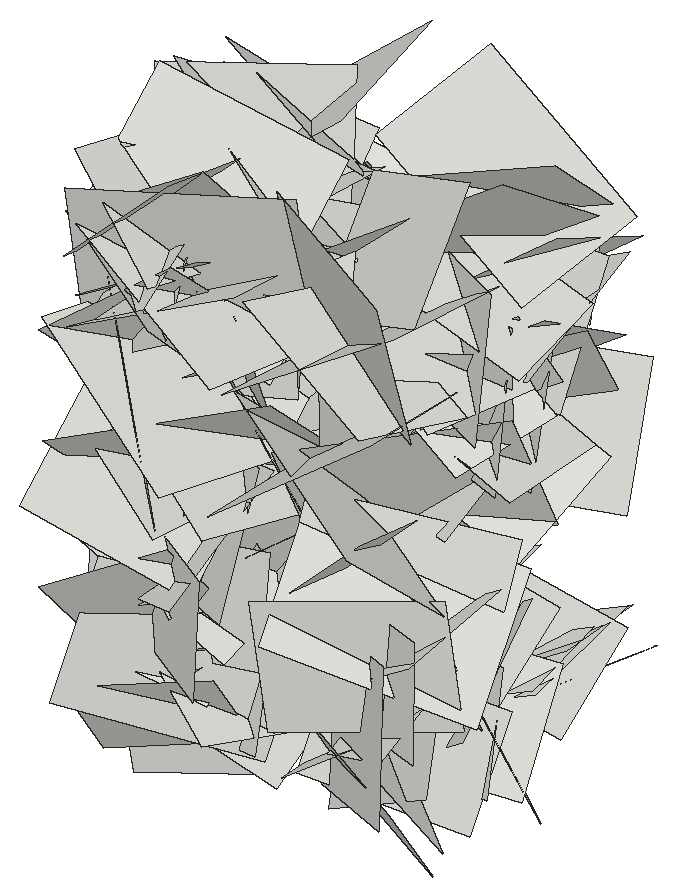
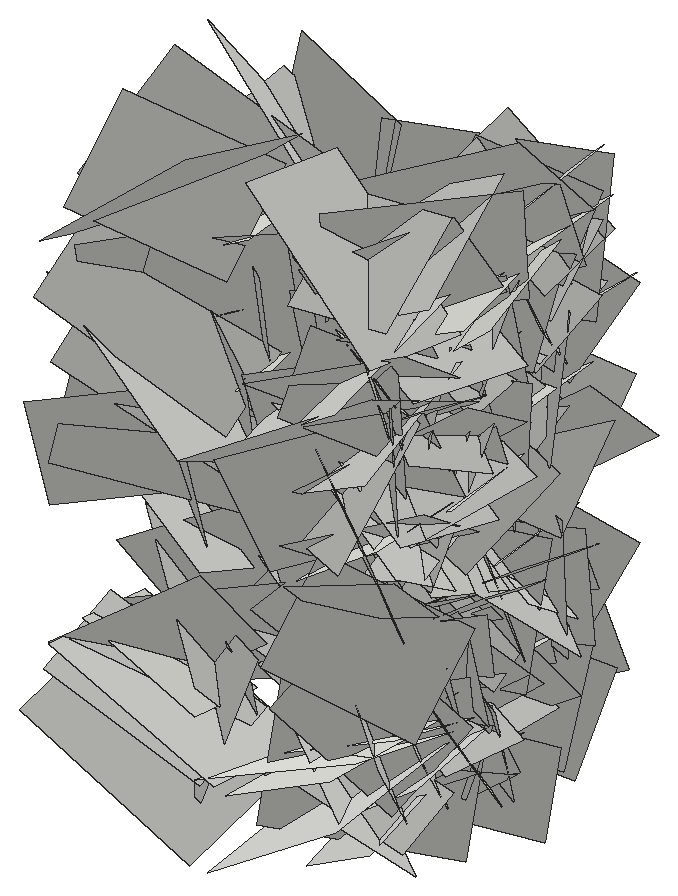
# SketchUp Ruby script. Lengths in inches.
U = 1.inch
M = Sketchup.active_model
def pt(a) = Geom::Point3d.new(a.map { |v| v * U })
def face(e, loops, mat)
  f = e.add_face(loops[0].map { |a| pt(a) })
  loops[1..].each { |l| e.add_face(l.map { |a| pt(a) }).erase! }
  f.material = f.back_material = mat if mat
  f
end
# faces: each face lists its corners as indices into pts; further lists are holes
def faces(e, pts, list, mat = nil) = list.each { |f| face(e, (f[0].is_a?(Array) ? f : [f]).map { |l| l.map { |i| pts[i] } }, mat) }
# xy, xz, yz: faces in a plane at the given z, y or x. An outline is a flat list of corners, or four numbers for a rectangle; further outlines are holes
def ring(l) = l.size == 4 ? [[l[0], l[1]], [l[2], l[1]], [l[2], l[3]], [l[0], l[3]]] : l.each_slice(2).to_a
def flat(e, list, mat, &to3) = list.each { |f| face(e, (f[0].is_a?(Array) ? f : [f]).map { |l| ring(l).map { |u, v| to3.(u, v) } }, mat) }
def xy(e, z, list, mat = nil) = flat(e, list, mat) { |x, y| [x, y, z] }
def xz(e, y, list, mat = nil) = flat(e, list, mat) { |x, z| [x, y, z] }
def yz(e, x, list, mat = nil) = flat(e, list, mat) { |y, z| [x, y, z] }
def lines(e, pts, list) = list.each { |a, b| e.add_line(pt(pts[a]), pt(pts[b])) }
# prism: a flat outline (further loops are holes) pulled along v
def prism(e, loops, v, mat = nil)
  f = face(e, loops, mat); d = Geom::Vector3d.new(v.map { |x| x * U })
  f.pushpull(f.normal.samedirection?(d) ? d.length : -d.length)
end
def box(e, o, s, mat = nil) = prism(e, [[o, [o[0] + s[0], o[1], o[2]], [o[0] + s[0], o[1] + s[1], o[2]], [o[0], o[1] + s[1], o[2]]]], [0, 0, s[2]], mat)
def at(x, y, z, deg = 0) = Geom::Transformation.translation(pt([x, y, z])) * Geom::Transformation.rotation(ORIGIN, Z_AXIS, deg.degrees)
def axes(o, x, y, z) = Geom::Transformation.new([*x, 0, *y, 0, *z, 0, *pt(o).to_a, 1])
def part(name) = M.definitions.add(name)
# library, detail: a bought-in or finely detailed component or shape, given as its bounding box
def library(name, o, s) = part(name).tap { |d| box(d.entities, o, s) }
def detail(e, o, s) = box(e.add_group.entities, o, s)
def put(e, d, t, mat = nil) = e.add_instance(d, t).tap { |i| i.material = mat if mat }
def group(e, t, mat = nil) = e.add_group.tap { |g| g.transformation = t; g.material = mat if mat }.entities
root = M.entities
c1 = part("Component\#6")
p = [[0.01,0,0],[0,3.24,4.54],[4.32,3.24,4.54],[4.33,0,0]]
faces(c1.entities,p,[[0,1,2,3]])
put(root,c1,axes([24.34,192.1875,23.6],[0.04344,0.89705,-0.17333],[-0.1764,-0.16328,-0.88435],[0.95226,-0.07116,-0.15591]))
put(root,c1,axes([28.31,192.1875,23.6],[-0.04344,0.89705,-0.17333],[0.1764,-0.16328,-0.88435],[-0.95226,-0.07116,-0.15591]))
put(root,c1,axes([24.34,200.85,9.74],[0.02518,0.49854,0.49521],[0.19267,0.47427,-0.48618],[0.7195,-0.14445,0.11286]))
put(root,c1,axes([28.31,200.46,4.14],[-0.03987,0.66432,-0.22968],[-0.12809,-0.2327,-0.65325],[-0.73398,0.00452,0.12648]))
put(root,c1,axes([24.34,196.11,19.5625],[-0.1708,0.27531,1.11719],[-0.21419,1.10379,-0.30115],[1.2007,0.23607,0.1052]))
put(root,c1,axes([24.34,195.27,-1.16],[-0.10176,-0.07093,0.82892],[0.16666,0.81783,0.08819],[0.86597,-0.16573,0.08043]))
put(root,c1,axes([28.31,202.11,15.27],[-0.00741,-0.76642,-0.19435],[-0.02033,-0.19414,0.76626],[-0.83787,0.01149,-0.01688]))
put(root,c1,axes([28.31,201.99,11.3125],[0.07595,0.62186,-0.76254],[0.14567,-0.76339,-0.60964],[-1.03278,-0.06194,-0.14206]))
put(root,c1,axes([24.34,202.38,16.09],[-0.07402,-0.92988,-0.45649],[-0.17154,-0.44211,0.92536],[1.08456,-0.13339,0.1152]))
put(root,c1,axes([24.34,193.92,18.08],[-0.13809,0.41624,-1.10581],[-0.27382,-1.09563,-0.38198],[1.22215,-0.19844,-0.21052]))
put(root,c1,axes([28.31,193.9,23.36],[-0.05376,0.55183,-0.55937],[0.04326,-0.55793,-0.55411],[-0.83178,-0.06469,0.00734]))
put(root,c1,axes([24.34,196.25,20.97],[0.03433,0.46285,-0.75346],[-0.09275,-0.74858,-0.46362],[0.93272,-0.09148,-0.01837]))
put(root,c1,axes([24.34,193.09,19.46],[0.07295,0.25641,0.83596],[-0.12348,0.83376,-0.24615],[0.9186,0.09171,-0.09948]))
put(root,c1,axes([28.31,200.69,6.875],[0.16125,-0.91938,-0.30199],[0.04119,-0.29965,0.93182],[-1.02494,-0.15668,-0.01006]))
put(root,c1,axes([24.34,194.43,21.03],[-0.18864,1.08922,-0.2367],[-0.12278,-0.25647,-1.09312],[1.17512,0.14806,-0.15221]))
put(root,c1,axes([24.34,195.95,14.86],[-0.17446,0.9838,0.62037],[-0.19333,0.59697,-0.99508],[1.2176,0.23574,-0.06911]))
put(root,c1,axes([24.34,200.41,3.58],[-0.05776,-0.87144,-0.04483],[0.06577,-0.04867,0.87073],[0.92261,-0.05109,-0.06488]))
put(root,c1,axes([24.34,198.3125,4.47],[-0.08144,0.93817,-0.09306],[-0.01009,-0.09413,-0.94116],[0.99929,0.07551,-0.01709]))
put(root,c1,axes([24.34,200.05,13.66],[0.07814,0.81604,-0.08962],[-0.02759,-0.08761,-0.81916],[0.86976,-0.0761,-0.01794]))
put(root,c1,axes([24.34,196.375,20.79],[-0.12547,0.87042,-0.10702],[0.18806,-0.08199,-0.86307],[0.91037,0.1369,0.16354]))
put(root,c1,axes([24.34,195.73,16.63],[-0.01219,-0.78698,0.32297],[0.05977,0.32158,0.78561],[0.89973,-0.03203,-0.04781]))
put(root,c1,axes([28.31,200.82,0.59],[-0.02153,-0.73416,-0.35765],[0.0933,-0.35764,0.72915],[-0.8606,-0.02041,0.08799]))
put(root,c1,axes([24.34,193.46,10.77],[0.10152,0.90556,-0.18731],[-0.17799,-0.16815,-0.89879],[0.96391,-0.12642,-0.14624]))
put(root,c1,axes([24.34,196.17,12.88],[-0.06274,0.02618,0.84664],[0.15393,0.83645,-0.01571],[0.88457,-0.1437,0.06278]))
put(root,c1,axes([24.34,195.4375,18.11],[0.16874,-0.51977,-0.57708],[-0.05885,-0.59519,0.52076],[0.82114,0.06415,0.15591]))
put(root,c1,axes([28.31,195.9375,9.16],[-0.07841,0.69576,-0.29748],[0.09095,-0.28926,-0.69787],[-0.79692,-0.10147,-0.05038]))
put(root,c1,axes([24.34,198.67,11.97],[-0.07539,0.76068,0.50866],[0.0723,0.51318,-0.75791],[0.96729,0.02092,0.0963]))
put(root,c1,axes([28.31,195.99,4.23],[0.18601,0.0566,0.88651],[-0.05201,0.90288,-0.04793],[-0.94017,-0.03875,0.17804]))
put(root,c1,axes([28.31,197.35,3.52],[-0.03443,0.41092,0.66217],[0.08038,0.66126,-0.40665],[-0.82215,0.04744,-0.06748]))
put(root,c1,axes([24.34,192.22,20.81],[0.00161,0.62306,-0.59539],[0.0785,-0.59329,-0.62067],[0.91013,0.05007,0.05459]))
put(root,c1,axes([28.31,202.74,-0.14],[-0.03158,-0.64507,0.25861],[-0.01592,0.25938,0.64528],[-0.73651,0.02205,-0.02503]))
put(root,c1,axes([24.34,195.86,16.68],[0.06531,-0.43873,0.684],[0.07025,0.68639,0.43429],[0.8585,-0.02279,-0.08757]))
put(root,c1,axes([28.31,202.51,19.98],[-0.06792,0.48446,-0.5602],[0.10116,-0.55221,-0.48846],[-0.77852,-0.11402,-0.01459]))
put(root,c1,axes([28.31,192.04,10.01],[0.12172,0.5206,-0.6372],[-0.01939,-0.6416,-0.52749],[-0.87198,0.08694,-0.07722]))
put(root,c1,axes([28.31,198.38,4.95],[0.02223,0.32868,-0.55446],[-0.17267,-0.53404,-0.32274],[-0.66105,0.15055,0.06565]))
put(root,c1,axes([24.34,199.37,10.67],[-0.09558,-1.01864,0.46326],[-0.13943,0.47118,1.01047],[1.17795,-0.02688,0.1572]))
put(root,c1,axes([28.31,192.95,10.8],[-0.02962,0.02518,0.78508],[0.12702,0.77652,-0.02064],[-0.82287,0.11896,-0.03145]))
put(root,c1,axes([28.31,200.03,9.27],[0.00412,-0.60297,0.30435],[-0.07057,0.30253,0.60022],[-0.71247,-0.03345,-0.05769]))
put(root,c1,axes([28.31,199.6875,17.84],[-0.07891,0.44569,0.39814],[-0.07493,0.39183,-0.45185],[-0.62903,-0.10259,0.00388]))
put(root,c1,axes([28.31,200.4375,8.06],[0.17377,0.75884,-0.49804],[0.05898,-0.51355,-0.76415],[-0.96033,0.10576,-0.13705]))
put(root,c1,axes([28.31,195.68,15.75],[-0.06715,-0.51242,0.33521],[-0.05381,0.34023,0.51051],[-0.64683,0.02489,-0.07727]))
put(root,c1,axes([28.31,198.91,12.75],[0.15355,-0.10183,1.00426],[0.21738,0.99636,0.07145],[-1.04766,0.19182,0.16201]))
put(root,c1,axes([28.31,196.5625,6.92],[-0.07674,-0.09799,-0.6482],[0.03176,-0.65195,0.09521],[-0.69417,-0.019,0.07601]))
put(root,c1,axes([28.31,199.23,1.1],[0.00098,-0.71414,-0.15761],[0.04174,-0.15733,0.71311],[-0.77408,-0.00939,0.03826]))
put(root,c1,axes([28.31,192.26,20.51],[0.14395,0.6641,-0.62024],[0.10915,-0.63433,-0.65665],[-0.95701,0.02754,-0.16819]))
put(root,c1,axes([28.31,193.91,15.9375],[-0.03263,0.61645,-0.26034],[0.02336,-0.25954,-0.61716],[-0.70894,-0.03692,-0.00835]))
put(root,c1,axes([28.31,202.9,8.46],[0.28421,-0.45126,-0.90988],[0.10984,-0.92399,0.48879],[-1.07096,-0.21452,-0.19133]))
put(root,c1,axes([24.34,199.68,18.17],[-0.10811,0.81171,0.57509],[0.11351,0.5837,-0.80488],[1.04835,0.0205,0.14645]))
put(root,c1,axes([28.31,193.57,4.75],[-0.0218,0.6351,0.02763],[-0.03876,0.02642,-0.63443],[-0.67273,-0.0221,0.03566]))
put(root,c1,axes([24.34,189.31,11.46],[0.01967,0.80876,0.77653],[-0.21901,0.76581,-0.79265],[1.16812,0.12996,-0.16169]))
put(root,c1,axes([24.34,202.76,13.17],[-0.11284,-1.03894,-0.17524],[0.03066,-0.17895,1.04335],[1.11641,-0.1001,-0.04636]))
put(root,c1,axes([28.31,195.85,11.01],[0.15114,0.73817,0.19544],[-0.07767,0.21113,-0.74396],[-0.80568,0.11812,0.10838]))
put(root,c1,axes([28.31,190.79,19.57],[-0.04866,0.55121,0.30162],[-0.00575,0.30207,-0.55285],[-0.66601,-0.04288,-0.01726]))
put(root,c1,axes([24.34,196.07,8.125],[0.08332,-0.69698,-0.457],[0.10667,-0.44773,0.70016],[0.87699,0.12068,-0.04174]))
put(root,c1,axes([28.31,199.64,2.06],[0.21894,0.61345,0.59822],[-0.01858,0.61825,-0.62794],[-0.90807,0.13525,0.15708]))
put(root,c1,axes([28.31,202.56,19.21],[-0.06396,-0.26998,-0.58675],[0.04641,-0.58965,0.26682],[-0.68306,-0.01478,0.07307]))
put(root,c1,axes([24.34,197.24,20.32],[0.11105,0.4932,0.81979],[-0.10012,0.82599,-0.48487],[1.00916,0.02768,-0.13831]))
put(root,c1,axes([24.34,196.19,13.89],[-0.03711,0.95345,-0.08325],[0.1071,-0.07916,-0.94908],[1.00884,0.04348,0.09769]))
put(root,c1,axes([28.31,198.53,13.8],[0.10676,-0.41647,0.70694],[0.09382,0.7136,0.40779],[-0.86465,0.02601,0.13154]))
put(root,c1,axes([28.31,201.03,8.02],[0.03451,-0.61291,-0.20918],[-0.0475,-0.21108,0.61149],[-0.68484,-0.01625,-0.05296]))
put(root,c1,axes([28.31,199.53,17.66],[0.07108,0.22718,0.77768],[0.14032,0.76678,-0.23541],[-0.84726,0.14605,0.02626]))
put(root,c1,axes([28.31,196.1,5.28],[0.08762,-0.56519,-0.39893],[-0.0287,-0.4041,0.56691],[-0.73275,-0.05175,-0.06991]))
put(root,c1,axes([24.34,192.44,8.79],[-0.05887,1.04295,0.25043],[0.00297,0.2509,-1.04431],[1.13694,0.05335,0.0157]))
put(root,c1,axes([24.34,193.71,0.46],[0.00413,-0.52236,0.7551],[0.18121,0.74232,0.51263],[0.95624,-0.13842,-0.10041]))
put(root,c1,axes([24.34,195.28,4.79],[0.03702,0.87634,0.85063],[-0.28559,0.83554,-0.84973],[1.26267,0.16329,-0.21713]))
put(root,c1,axes([24.34,203.91,5.3125],[0.18463,-0.58129,-0.78091],[-0.13848,-0.80009,0.56643],[1.02258,-0.00339,0.2177]))
put(root,c1,axes([24.34,198.93,5.125],[0.08676,0.85287,0.14934],[0.16568,0.13299,-0.84515],[0.90272,-0.10637,0.14076]))
put(root,c1,axes([24.34,198.84,9.75],[-0.24721,-0.9594,-0.88495],[-0.06038,-0.89063,0.98057],[1.38221,-0.2105,-0.11544]))
put(root,c1,axes([24.34,202.1,18.26],[-0.1919,-1.13475,-0.09678],[0.16378,-0.12156,1.13628],[1.19604,-0.16542,-0.17113]))
put(root,c1,axes([28.31,194.11,10.49],[0.01019,-0.66626,0.06574],[0.1187,0.06642,0.65679],[-0.69967,0.00157,0.11238]))
put(root,c1,axes([24.34,200.51,5.45],[-0.07717,-0.59417,-0.91785],[0.09928,-0.91989,0.58806],[1.15472,0.03938,-0.1119]))
put(root,c1,axes([24.34,205.24,14.9],[-0.1168,-0.46047,-1.13614],[-0.0362,-1.13913,0.465],[1.29896,-0.07315,-0.0892]))
put(root,c1,axes([24.34,194.25,1.05],[0.1707,-0.55728,0.79671],[-0.04122,0.80323,0.5697],[1.02978,0.12452,-0.10926]))
put(root,c1,axes([24.34,194.35,10.5],[-0.1187,0.07765,-1.12146],[0.14385,-1.11784,-0.09095],[1.18288,0.14373,-0.10148]))
put(root,c1,axes([24.34,197.36,24.8],[-0.09794,1.0389,-0.68546],[-0.01654,-0.68826,-1.04104],[1.31923,0.0685,-0.06394]))
put(root,c1,axes([28.31,199.74,12.37],[0.13977,-0.41949,-0.41774],[-0.0557,-0.43458,0.41982],[-0.62506,-0.05508,-0.13082]))
put(root,c1,axes([28.31,199.42,15.6],[0.03605,-0.49998,-0.38134],[0.14474,-0.36691,0.49324],[-0.65063,-0.10932,0.0886]))
put(root,c1,axes([24.34,200.08,24.34],[0.03463,0.75517,-0.67877],[0.20748,-0.67107,-0.73718],[1.05612,0.10708,0.16708]))
put(root,c1,axes([24.34,199.09,16.39],[0.13116,-1.14374,0.05938],[-0.13174,0.04596,1.1443],[1.20683,0.12933,0.11846]))
put(root,c1,axes([24.34,192.66,5.0625],[0.03803,0.06475,1.02957],[0.25075,1.00223,-0.07127],[1.06436,-0.23842,-0.02]))
put(root,c1,axes([24.34,196.53,2.03],[0.14871,0.38131,0.94323],[0.09041,0.94439,-0.39446],[1.07463,-0.13222,-0.09734]))
put(root,c1,axes([24.34,200.2,14.91],[0.20407,-0.96139,-0.18597],[0.07393,-0.17559,0.97991],[1.03533,0.20204,-0.03331]))
put(root,c1,axes([24.34,198.375,11.05],[-0.00636,-0.47599,-1.14741],[-0.03555,-1.14695,0.47597],[1.31628,-0.03327,0.00731]))
put(root,c1,axes([24.34,202.25,12.93],[-0.19135,-1.27912,0.12446],[0.2118,0.09622,1.27869],[1.34571,-0.19703,-0.18355]))
put(root,c1,axes([24.34,197.86,18.23],[0.19608,0.2602,-1.0463],[-0.01915,-1.06069,-0.26697],[1.14269,-0.06243,0.17507]))
put(root,c1,axes([24.34,197.84,4.84],[0.11369,-0.36766,-0.96616],[0.19069,-0.94989,0.38144],[1.07906,0.2066,0.03439]))
put(root,c1,axes([24.34,200.375,7.61],[0.26418,-0.51362,-0.84712],[0.05211,-0.86603,0.53955],[1.04881,0.1724,0.18657]))
put(root,c1,axes([24.34,203.04,12.11],[0.14841,-0.94408,-0.5752],[0.05434,-0.57362,0.95398],[1.17058,0.14632,0.02864]))
put(root,c1,axes([24.34,199.56,18.73],[0.07364,1.07871,-0.62029],[-0.05176,-0.61841,-1.08091],[1.31797,-0.08456,-0.00779]))
put(root,c1,axes([24.34,204.42,20.53],[0.1154,-1.25003,-0.28156],[-0.14973,-0.29256,1.24425],[1.34995,0.07441,0.16208]))
put(root,c1,axes([24.34,195.93,15.54],[0.04965,0.25406,1.2028],[0.02984,1.20314,-0.25523],[1.30276,-0.03724,-0.03999]))
put(root,c1,axes([24.34,198.85,12.57],[0.15345,0.48368,1.12599],[-0.09378,1.13498,-0.47617],[1.29562,0.02486,-0.16783]))
put(root,c1,axes([24.34,200.7,5.85],[0.20906,1.0682,-0.14016],[0.07965,-0.15578,-1.08152],[1.13921,-0.18514,0.10133]))
put(root,c1,axes([24.34,194.09,6.34],[0.25898,1.07168,-0.21064],[-0.01285,-0.21318,-1.09862],[1.15764,-0.24212,0.03493]))
put(root,c1,axes([24.34,192.7,21.39],[0.08893,0.79245,0.9015],[0.06254,0.89988,-0.79652],[1.27076,-0.09974,-0.02389]))
put(root,c1,axes([24.34,199.38,-0.0625],[0.15183,-0.50198,1.07326],[0.00307,1.08122,0.50532],[1.25594,0.05804,-0.13098]))
put(root,c1,axes([24.34,200.25,4.79],[0.06637,1.27776,-0.24675],[-0.01199,-0.2465,-1.2793],[1.3794,-0.06362,0.00075]))
put(root,c1,axes([24.34,192.73,15.73],[0.12897,1.2724,-0.23633],[-0.08155,-0.22984,-1.27707],[1.36939,-0.13352,-0.05379]))
put(root,c1,axes([24.34,200.21,21.54],[0.14018,1.21556,-0.55877],[-0.14242,-0.54659,-1.22085],[1.41094,-0.17594,-0.06772]))
put(root,c1,axes([24.34,190.45,18.05],[0.16537,1.24759,-0.14593],[-0.05265,-0.14081,-1.25691],[1.33042,-0.16065,-0.0316]))
put(root,c1,axes([24.34,190.86,3.39],[0.21383,0.32739,1.20741],[-0.09698,1.22359,-0.31649],[1.32251,0.03679,-0.21843]))
put(root,c1,axes([24.34,195.52,16.87],[0.17814,-1.09516,0.21581],[0.19304,0.24222,1.08736],[1.16734,0.12707,-0.21275]))
put(root,c1,axes([24.34,201.79,17.38],[0.19939,0.73728,-1.06028],[-0.09629,-1.06126,-0.75408],[1.36551,-0.18249,0.10164]))
put(root,c1,axes([24.34,196.26,4.8],[0.10051,-0.43998,1.12809],[0.21352,1.12151,0.42048],[1.26562,-0.15427,-0.16053]))
put(root,c1,axes([24.34,191.67,21.5],[0.0579,1.33618,-0.15223],[0.05318,-0.15428,-1.33612],[1.42453,-0.04855,0.05606]))
put(root,c1,axes([24.34,198.6875,16.83],[0.02201,1.26014,0.56955],[0.0456,0.56875,-1.25994],[1.46513,-0.03663,0.03065]))
put(root,c1,axes([24.34,196.95,13.22],[0.12152,0.35472,1.26895],[0.01769,1.27325,-0.35743],[1.39654,-0.047,-0.10589]))
put(root,c1,axes([24.34,197.84,15.77],[0.08558,0.66637,-1.22765],[0.01617,-1.23004,-0.66667],[1.48057,-0.02508,0.07824]))
put(root,c1,axes([24.34,193.34,3.5],[0.3285,0.68164,0.95344],[0.04901,0.97833,-0.71446],[1.2414,-0.219,-0.22409]))
put(root,c1,axes([24.34,192.59,17.15],[0.08597,-0.32374,1.28455],[0.18245,1.27862,0.31138],[1.3923,-0.14756,-0.12012]))
put(root,c1,axes([24.34,199.09,4.9],[0.11121,1.25407,0.182],[0.25083,0.16003,-1.23904],[1.31962,-0.1361,0.22018]))
put(root,c1,axes([24.34,194.4,9.86],[0.11876,-1.04596,0.91618],[0.1474,0.92297,1.03671],[1.46651,-0.00807,-0.1784]))
put(root,c1,axes([24.34,202.95,19.72],[0.19445,-0.3512,-1.29554],[0.25274,-1.27827,0.38028],[1.40021,0.2795,0.11127]))
put(root,c1,axes([38.11,202.95,19.72],[-0.19445,-0.3512,-1.29554],[-0.25274,-1.27827,0.38028],[-1.40021,0.2795,0.11127]))
put(root,c1,axes([38.11,194.4,9.86],[-0.11876,-1.04596,0.91618],[-0.1474,0.92297,1.03671],[-1.46651,-0.00807,-0.1784]))
put(root,c1,axes([38.11,199.09,4.9],[-0.11121,1.25407,0.182],[-0.25083,0.16003,-1.23904],[-1.31962,-0.1361,0.22018]))
put(root,c1,axes([38.11,192.59,17.15],[-0.08597,-0.32374,1.28455],[-0.18245,1.27862,0.31138],[-1.3923,-0.14756,-0.12012]))
put(root,c1,axes([38.11,193.34,3.5],[-0.3285,0.68164,0.95344],[-0.04901,0.97833,-0.71446],[-1.2414,-0.219,-0.22409]))
put(root,c1,axes([38.11,197.84,15.77],[-0.08558,0.66637,-1.22765],[-0.01617,-1.23004,-0.66667],[-1.48057,-0.02508,0.07824]))
put(root,c1,axes([38.11,196.95,13.22],[-0.12152,0.35472,1.26895],[-0.01769,1.27325,-0.35743],[-1.39654,-0.047,-0.10589]))
put(root,c1,axes([38.11,198.6875,16.83],[-0.02201,1.26014,0.56955],[-0.0456,0.56875,-1.25994],[-1.46513,-0.03663,0.03065]))
put(root,c1,axes([38.11,191.67,21.5],[-0.0579,1.33618,-0.15223],[-0.05318,-0.15428,-1.33612],[-1.42453,-0.04855,0.05606]))
put(root,c1,axes([38.11,196.26,4.8],[-0.10051,-0.43998,1.12809],[-0.21352,1.12151,0.42048],[-1.26562,-0.15427,-0.16053]))
put(root,c1,axes([38.11,201.79,17.38],[-0.19939,0.73728,-1.06028],[0.09629,-1.06126,-0.75408],[-1.36551,-0.18249,0.10164]))
put(root,c1,axes([38.11,195.52,16.87],[-0.17814,-1.09516,0.21581],[-0.19304,0.24222,1.08736],[-1.16734,0.12707,-0.21275]))
put(root,c1,axes([38.11,190.86,3.39],[-0.21383,0.32739,1.20741],[0.09698,1.22359,-0.31649],[-1.32251,0.03679,-0.21843]))
put(root,c1,axes([38.11,190.45,18.05],[-0.16537,1.24759,-0.14593],[0.05265,-0.14081,-1.25691],[-1.33042,-0.16065,-0.0316]))
put(root,c1,axes([38.11,200.21,21.54],[-0.14018,1.21556,-0.55877],[0.14242,-0.54659,-1.22085],[-1.41094,-0.17594,-0.06772]))
put(root,c1,axes([38.11,192.73,15.73],[-0.12897,1.2724,-0.23633],[0.08155,-0.22984,-1.27707],[-1.36939,-0.13352,-0.05379]))
put(root,c1,axes([38.11,200.25,4.79],[-0.06637,1.27776,-0.24675],[0.01199,-0.2465,-1.2793],[-1.3794,-0.06362,0.00075]))
put(root,c1,axes([38.11,199.38,-0.0625],[-0.15183,-0.50198,1.07326],[-0.00307,1.08122,0.50532],[-1.25594,0.05804,-0.13098]))
put(root,c1,axes([38.11,192.7,21.39],[-0.08893,0.79245,0.9015],[-0.06254,0.89988,-0.79652],[-1.27076,-0.09974,-0.02389]))
put(root,c1,axes([38.11,194.09,6.34],[-0.25898,1.07168,-0.21064],[0.01285,-0.21318,-1.09862],[-1.15764,-0.24212,0.03493]))
put(root,c1,axes([38.11,200.7,5.85],[-0.20906,1.0682,-0.14016],[-0.07965,-0.15578,-1.08152],[-1.13921,-0.18514,0.10133]))
put(root,c1,axes([38.11,198.85,12.57],[-0.15345,0.48368,1.12599],[0.09378,1.13498,-0.47617],[-1.29562,0.02486,-0.16783]))
put(root,c1,axes([38.11,195.93,15.54],[-0.04965,0.25406,1.2028],[-0.02984,1.20314,-0.25523],[-1.30276,-0.03724,-0.03999]))
put(root,c1,axes([38.11,204.42,20.53],[-0.1154,-1.25003,-0.28156],[0.14973,-0.29256,1.24425],[-1.34995,0.07441,0.16208]))
put(root,c1,axes([38.11,199.56,18.73],[-0.07364,1.07871,-0.62029],[0.05176,-0.61841,-1.08091],[-1.31797,-0.08456,-0.00779]))
put(root,c1,axes([38.11,203.04,12.11],[-0.14841,-0.94408,-0.5752],[-0.05434,-0.57362,0.95398],[-1.17058,0.14632,0.02864]))
put(root,c1,axes([38.11,200.375,7.61],[-0.26418,-0.51362,-0.84712],[-0.05211,-0.86603,0.53955],[-1.04881,0.1724,0.18657]))
put(root,c1,axes([38.11,197.84,4.84],[-0.11369,-0.36766,-0.96616],[-0.19069,-0.94989,0.38144],[-1.07906,0.2066,0.03439]))
put(root,c1,axes([38.11,197.86,18.23],[-0.19608,0.2602,-1.0463],[0.01915,-1.06069,-0.26697],[-1.14269,-0.06243,0.17507]))
put(root,c1,axes([38.11,202.25,12.93],[0.19135,-1.27912,0.12446],[-0.2118,0.09622,1.27869],[-1.34571,-0.19703,-0.18355]))
put(root,c1,axes([38.11,198.375,11.05],[0.00636,-0.47599,-1.14741],[0.03555,-1.14695,0.47597],[-1.31628,-0.03327,0.00731]))
put(root,c1,axes([38.11,200.2,14.91],[-0.20407,-0.96139,-0.18597],[-0.07393,-0.17559,0.97991],[-1.03533,0.20204,-0.03331]))
put(root,c1,axes([38.11,196.53,2.03],[-0.14871,0.38131,0.94323],[-0.09041,0.94439,-0.39446],[-1.07463,-0.13222,-0.09734]))
put(root,c1,axes([38.11,192.66,5.0625],[-0.03803,0.06475,1.02957],[-0.25075,1.00223,-0.07127],[-1.06436,-0.23842,-0.02]))
put(root,c1,axes([38.11,199.09,16.39],[-0.13116,-1.14374,0.05938],[0.13174,0.04596,1.1443],[-1.20683,0.12933,0.11846]))
put(root,c1,axes([38.11,200.08,24.34],[-0.03463,0.75517,-0.67877],[-0.20748,-0.67107,-0.73718],[-1.05612,0.10708,0.16708]))
put(root,c1,axes([34.14,199.42,15.6],[-0.03605,-0.49998,-0.38134],[-0.14474,-0.36691,0.49324],[0.65063,-0.10932,0.0886]))
put(root,c1,axes([34.14,199.74,12.37],[-0.13977,-0.41949,-0.41774],[0.0557,-0.43458,0.41982],[0.62506,-0.05508,-0.13082]))
put(root,c1,axes([38.11,197.36,24.8],[0.09794,1.0389,-0.68546],[0.01654,-0.68826,-1.04104],[-1.31923,0.0685,-0.06394]))
put(root,c1,axes([38.11,194.35,10.5],[0.1187,0.07765,-1.12146],[-0.14385,-1.11784,-0.09095],[-1.18288,0.14373,-0.10148]))
put(root,c1,axes([38.11,194.25,1.05],[-0.1707,-0.55728,0.79671],[0.04122,0.80323,0.5697],[-1.02978,0.12452,-0.10926]))
put(root,c1,axes([38.11,205.24,14.9],[0.1168,-0.46047,-1.13614],[0.0362,-1.13913,0.465],[-1.29896,-0.07315,-0.0892]))
put(root,c1,axes([38.11,200.51,5.45],[0.07717,-0.59417,-0.91785],[-0.09928,-0.91989,0.58806],[-1.15472,0.03938,-0.1119]))
put(root,c1,axes([34.14,194.11,10.49],[-0.01019,-0.66626,0.06574],[-0.1187,0.06642,0.65679],[0.69967,0.00157,0.11238]))
put(root,c1,axes([38.11,202.1,18.26],[0.1919,-1.13475,-0.09678],[-0.16378,-0.12156,1.13628],[-1.19604,-0.16542,-0.17113]))
put(root,c1,axes([38.11,198.84,9.75],[0.24721,-0.9594,-0.88495],[0.06038,-0.89063,0.98057],[-1.38221,-0.2105,-0.11544]))
put(root,c1,axes([38.11,198.93,5.125],[-0.08676,0.85287,0.14934],[-0.16568,0.13299,-0.84515],[-0.90272,-0.10637,0.14076]))
put(root,c1,axes([38.11,203.91,5.3125],[-0.18463,-0.58129,-0.78091],[0.13848,-0.80009,0.56643],[-1.02258,-0.00339,0.2177]))
put(root,c1,axes([38.11,195.28,4.79],[-0.03702,0.87634,0.85063],[0.28559,0.83554,-0.84973],[-1.26267,0.16329,-0.21713]))
put(root,c1,axes([38.11,193.71,0.46],[-0.00413,-0.52236,0.7551],[-0.18121,0.74232,0.51263],[-0.95624,-0.13842,-0.10041]))
put(root,c1,axes([38.11,192.44,8.79],[0.05887,1.04295,0.25043],[-0.00297,0.2509,-1.04431],[-1.13694,0.05335,0.0157]))
put(root,c1,axes([34.14,196.1,5.28],[-0.08762,-0.56519,-0.39893],[0.0287,-0.4041,0.56691],[0.73275,-0.05175,-0.06991]))
put(root,c1,axes([34.14,199.53,17.66],[-0.07108,0.22718,0.77768],[-0.14032,0.76678,-0.23541],[0.84726,0.14605,0.02626]))
put(root,c1,axes([34.14,201.03,8.02],[-0.03451,-0.61291,-0.20918],[0.0475,-0.21108,0.61149],[0.68484,-0.01625,-0.05296]))
put(root,c1,axes([34.14,198.53,13.8],[-0.10676,-0.41647,0.70694],[-0.09382,0.7136,0.40779],[0.86465,0.02601,0.13154]))
